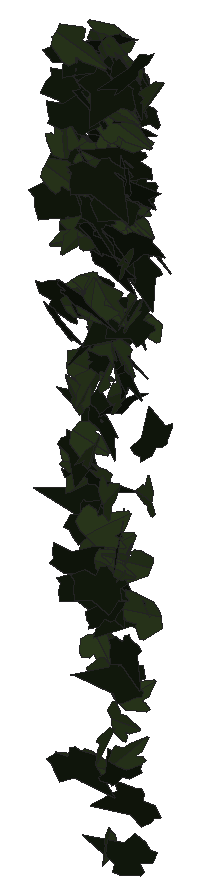
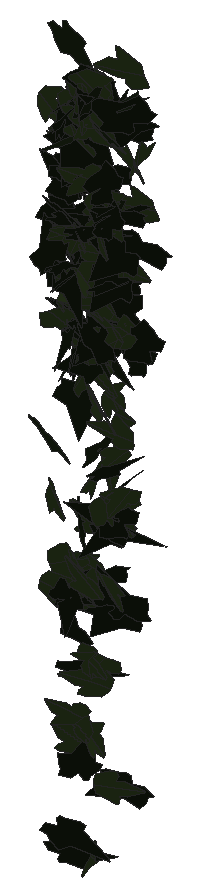
# SketchUp Ruby script. Lengths in inches.
U = 1.inch
M = Sketchup.active_model
def pt(a) = Geom::Point3d.new(a.map { |v| v * U })
def face(e, loops, mat)
  f = e.add_face(loops[0].map { |a| pt(a) })
  loops[1..].each { |l| e.add_face(l.map { |a| pt(a) }).erase! }
  f.material = f.back_material = mat if mat
  f
end
# faces: each face lists its corners as indices into pts; further lists are holes
def faces(e, pts, list, mat = nil) = list.each { |f| face(e, (f[0].is_a?(Array) ? f : [f]).map { |l| l.map { |i| pts[i] } }, mat) }
# xy, xz, yz: faces in a plane at the given z, y or x. An outline is a flat list of corners, or four numbers for a rectangle; further outlines are holes
def ring(l) = l.size == 4 ? [[l[0], l[1]], [l[2], l[1]], [l[2], l[3]], [l[0], l[3]]] : l.each_slice(2).to_a
def flat(e, list, mat, &to3) = list.each { |f| face(e, (f[0].is_a?(Array) ? f : [f]).map { |l| ring(l).map { |u, v| to3.(u, v) } }, mat) }
def xy(e, z, list, mat = nil) = flat(e, list, mat) { |x, y| [x, y, z] }
def xz(e, y, list, mat = nil) = flat(e, list, mat) { |x, z| [x, y, z] }
def yz(e, x, list, mat = nil) = flat(e, list, mat) { |y, z| [x, y, z] }
def lines(e, pts, list) = list.each { |a, b| e.add_line(pt(pts[a]), pt(pts[b])) }
# prism: a flat outline (further loops are holes) pulled along v
def prism(e, loops, v, mat = nil)
  f = face(e, loops, mat); d = Geom::Vector3d.new(v.map { |x| x * U })
  f.pushpull(f.normal.samedirection?(d) ? d.length : -d.length)
end
def box(e, o, s, mat = nil) = prism(e, [[o, [o[0] + s[0], o[1], o[2]], [o[0] + s[0], o[1] + s[1], o[2]], [o[0], o[1] + s[1], o[2]]]], [0, 0, s[2]], mat)
def at(x, y, z, deg = 0) = Geom::Transformation.translation(pt([x, y, z])) * Geom::Transformation.rotation(ORIGIN, Z_AXIS, deg.degrees)
def axes(o, x, y, z) = Geom::Transformation.new([*x, 0, *y, 0, *z, 0, *pt(o).to_a, 1])
def part(name) = M.definitions.add(name)
# library, detail: a bought-in or finely detailed component or shape, given as its bounding box
def library(name, o, s) = part(name).tap { |d| box(d.entities, o, s) }
def detail(e, o, s) = box(e.add_group.entities, o, s)
def put(e, d, t, mat = nil) = e.add_instance(d, t).tap { |i| i.material = mat if mat }
def group(e, t, mat = nil) = e.add_group.tap { |g| g.transformation = t; g.material = mat if mat }.entities
root = M.entities
M.materials.add("1026 AP 7946 SUNNY SIDE UP").color = [254, 231, 186]
M.materials.add("efeu1").color = [18, 25, 13]
M.materials.add("efeu2").color = [43, 57, 29]
c1 = part("ivyleaf_9")
p = [[1.54,2.16,1.25],[1.36,2.04,1.19],[-0.21,0.99,0.68],[-0.71,1.11,0.82],[-0.85,0.86,0.67],[-0.8,0.17,0.21],
  [-0.9,-0.01,0.1],[-0.67,-0.16,-0.02],[-0.08,-0.08,-0.05],[-0.03,-0.6,-0.4],[0.65,-0.88,-0.66],[0.83,-0.6,-0.49],
  [1.29,-0.42,-0.43],[1.8125,-0.07,-0.26],[1.21,0.44,0.15]]
faces(c1.entities,p,[[0,1,2,3,4,5,6,7,8,9,10,11,12,13,14]],"efeu1")
c2 = part("ivyleaf_10")
p = [[0,0.5,-0.03],[-0.0625,2.02,-0.43],[-0.19,2.01,-0.46],[-0.54,1.05,-0.29],[-0.52,0.625,-0.18],[-0.83,0.76,-0.28],
  [-1.16,0.64,-0.33],[-1.15,0.33,-0.24],[-0.77,-0.39,0.02],[-0.3,-0.51,0.16],[0.04,-0.48,0.23],[-0.02,2.01,-0.4375],
  [-0.06,2.01,-0.43],[0.04,-0.49,0.23],[0.67,-0.49,0.14],[1.38,0.36,-0.2],[1.375,0.51,-0.24],[0.81,0.65,-0.19],
  [0.62,0.59,-0.15],[0.6,1.09,-0.28],[0.5,1.23,-0.31]]
faces(c2.entities,p,[[0,1,2,3,4,5,6,7,8,9,10],[11,12,0,13,14,15,16,17,18,19,20]],"efeu2")
put(root,c1,axes([117.72,211.5625,267.85],[-0.26724,0.28496,-0.02816],[0.00004,-0.03365,-0.34156],[-0.45038,-0.16909,0.01668]),"1026 AP 7946 SUNNY SIDE UP")
put(root,c1,axes([116.79,211.63,257.41],[-0.02076,-0.2244,-0.18737],[0.03062,0.17968,-0.23041],[0.45189,-0.02249,0.00701]),"1026 AP 7946 SUNNY SIDE UP")
put(root,c2,axes([116.09,211.51,265.79],[-0.01025,0.27119,-0.1331],[-0.00358,0.13072,0.28022],[0.47338,0.00686,-0.00077]),"1026 AP 7946 SUNNY SIDE UP")
put(root,c1,axes([116.12,211.68,262.83],[0.32105,-0.12024,0.12963],[0.15877,-0.07745,-0.24415],[0.22386,0.22737,-0.01276]),"1026 AP 7946 SUNNY SIDE UP")
put(root,c2,axes([117.15,211.84,261.14],[-0.07556,0.10256,0.29182],[0.18442,-0.2572,0.11517],[0.43539,0.12674,0.00186]),"1026 AP 7946 SUNNY SIDE UP")
put(root,c2,axes([117.125,211.43,259.16],[0.0733,-0.01867,-0.30202],[0.03099,0.29626,-0.01448],[0.46071,-0.01696,0.04903]),"1026 AP 7946 SUNNY SIDE UP")
put(root,c1,axes([117.27,211.76,256.19],[-0.12056,-0.04186,-0.24779],[0.38238,0.00622,-0.08102],[0.02944,-0.25215,0.03762]),"1026 AP 7946 SUNNY SIDE UP")
put(root,c1,axes([116.625,211.8,264.67],[0.12053,-0.26928,0.01514],[-0.00287,-0.01738,-0.28845],[0.42417,0.0764,-0.00626]),"1026 AP 7946 SUNNY SIDE UP")
put(root,c1,axes([116.74,211.69,265.49],[-0.06701,-0.22295,-0.2213],[0.09219,0.20581,-0.23221],[0.47661,-0.07116,0.0138]),"1026 AP 7946 SUNNY SIDE UP")
put(root,c1,axes([116.25,211.62,266.28],[-0.25433,-0.035,0.20143],[0.29964,0.04473,0.17073],[-0.08923,0.24994,-0.00081]),"1026 AP 7946 SUNNY SIDE UP")
put(root,c1,axes([117.07,211.52,256.78],[-0.30564,0.1542,-0.11242],[-0.11394,0.08508,0.25529],[0.27517,0.2065,-0.01915]),"1026 AP 7946 SUNNY SIDE UP")
put(root,c2,axes([116.74,211.63,258.34],[0.32859,0.02524,-0.21949],[0.32306,0.0628,0.21549],[0.09792,-0.29186,0.02559]),"1026 AP 7946 SUNNY SIDE UP")
put(root,c1,axes([117.26,211.88,261.42],[0.01288,0.043,0.27915],[-0.13755,-0.25628,0.04316],[0.40849,-0.08765,0.00573]),"1026 AP 7946 SUNNY SIDE UP")
put(root,c2,axes([117.11,211.83,261.97],[-0.13057,0.05799,-0.24048],[0.22672,-0.18609,-0.10141],[-0.30335,-0.16404,0.02772]),"1026 AP 7946 SUNNY SIDE UP")
put(root,c2,axes([116.46,211.89,261.13],[-0.02177,-0.18039,0.2002],[0.07607,-0.19407,-0.18221],[0.41113,0.02636,0.04431]),"1026 AP 7946 SUNNY SIDE UP")
put(root,c1,axes([117.25,211.66,261.83],[0.26321,-0.14179,-0.16578],[-0.19682,0.09992,-0.22538],[0.27268,0.20898,-0.00265]),"1026 AP 7946 SUNNY SIDE UP")
put(root,c1,axes([117.39,211.66,264.42],[0.34811,0.14712,-0.16273],[-0.18976,-0.10467,-0.27386],[-0.28257,0.25154,-0.01656]),"1026 AP 7946 SUNNY SIDE UP")
put(root,c2,axes([115.73,211.74,265.09],[0.118,0.0225,0.25752],[0.39046,0.03029,-0.07948],[-0.05589,0.2591,-0.01152]),"1026 AP 7946 SUNNY SIDE UP")
put(root,c2,axes([116.88,211.87,254.21],[0.07301,-0.22861,0.12838],[0.04624,-0.12249,-0.241],[0.40777,0.05482,0.00434]),"1026 AP 7946 SUNNY SIDE UP")
put(root,c1,axes([115.6875,211.88,262.07],[0.13236,-0.1288,0.1951],[0.14711,-0.16568,-0.15928],[0.32975,0.12561,-0.00725]),"1026 AP 7946 SUNNY SIDE UP")
put(root,c1,axes([116.75,211.7,264.22],[0.41584,-0.01644,-0.15846],[-0.24309,-0.02609,-0.27128],[0.00162,0.30478,-0.02997]),"1026 AP 7946 SUNNY SIDE UP")
put(root,c1,axes([117.06,211.97,258.49],[-0.13244,0.00523,-0.31244],[0.40971,-0.15995,-0.07832],[-0.24427,-0.27112,0.03803]),"1026 AP 7946 SUNNY SIDE UP")
put(root,c1,axes([116.96,211.91,267.13],[-0.38473,-0.10593,-0.05945],[0.09598,0.00225,-0.27375],[0.16307,-0.25124,0.02088]),"1026 AP 7946 SUNNY SIDE UP")
put(root,c2,axes([117.38,211.86,264.01],[0.07415,-0.2657,0.03557],[0.0027,-0.03629,-0.27817],[0.42161,0.04696,-0.00447]),"1026 AP 7946 SUNNY SIDE UP")
put(root,c2,axes([116.57,211.76,262.6],[0.41928,-0.03942,0.02358],[-0.02972,0.02947,0.27653],[-0.06542,-0.26602,0.02553]),"1026 AP 7946 SUNNY SIDE UP")
put(root,c2,axes([116.38,211.72,260.71],[0.18063,-0.02954,0.22912],[-0.31798,0.09502,0.12107],[-0.1534,-0.23175,0.01883]),"1026 AP 7946 SUNNY SIDE UP")
put(root,c2,axes([115.94,211.82,267.76],[0.13322,0.02536,0.31168],[0.47296,0.03459,-0.0896],[-0.06324,0.31214,-0.01354]),"1026 AP 7946 SUNNY SIDE UP")
put(root,c1,axes([117.33,211.94,255.38],[-0.24724,-0.01,0.22267],[-0.32651,-0.06836,-0.15924],[0.09593,-0.25844,0.03188]),"1026 AP 7946 SUNNY SIDE UP")
put(root,c2,axes([116.74,211.9,257.58],[0.00141,-0.02321,-0.26083],[0.35543,-0.11553,0.01107],[-0.18254,-0.22514,0.01953]),"1026 AP 7946 SUNNY SIDE UP")
put(root,c1,axes([116.07,211.8,253.49],[-0.0324,-0.06753,-0.25995],[0.27629,0.18319,-0.06432],[0.30313,-0.17419,0.03084]),"1026 AP 7946 SUNNY SIDE UP")
put(root,c1,axes([117.2,212,256.84],[-0.34404,-0.14638,0.03912],[-0.02925,-0.04169,-0.27031],[0.23631,-0.21827,0.0235]),"1026 AP 7946 SUNNY SIDE UP")
put(root,c2,axes([116.7,211.875,262.91],[0.24586,0.01335,0.2242],[0.34266,-0.00423,-0.16111],[-0.00685,0.26788,-0.01214]),"1026 AP 7946 SUNNY SIDE UP")
put(root,c1,axes([117.11,211.93,253.45],[0.17044,0.1016,0.21229],[-0.27357,-0.11155,0.15071],[0.23471,-0.2038,0.0215]),"1026 AP 7946 SUNNY SIDE UP")
put(root,c2,axes([117.26,211.75,253.9],[-0.08504,-0.19327,0.17992],[0.04972,0.17331,0.20739],[-0.40774,0.06144,-0.01223]),"1026 AP 7946 SUNNY SIDE UP")
put(root,c2,axes([115.97,211.8,265.82],[0.3706,-0.14862,0.05043],[-0.04277,0.04978,0.28597],[-0.24271,-0.2357,0.02661]),"1026 AP 7946 SUNNY SIDE UP")
put(root,c2,axes([116.52,211.83,259.81],[-0.00742,-0.25742,-0.07225],[-0.00589,0.06874,-0.26479],[0.41889,-0.00359,-0.005]),"1026 AP 7946 SUNNY SIDE UP")
put(root,c1,axes([116.43,212.03,266.51],[0.22781,-0.24043,-0.04475],[0.05576,-0.02768,0.28855],[-0.37972,-0.14831,0.01552]),"1026 AP 7946 SUNNY SIDE UP")
put(root,c1,axes([115.6,211.92,262.4],[0.13012,-0.03081,0.27194],[0.34334,-0.15004,-0.08938],[0.23869,0.23261,-0.01968]),"1026 AP 7946 SUNNY SIDE UP")
put(root,c1,axes([116.41,211.71,258.5],[0.07428,-0.06146,-0.28555],[-0.10241,0.2708,-0.0718],[0.43398,0.07442,0.03193]),"1026 AP 7946 SUNNY SIDE UP")
put(root,c1,axes([116.95,212.07,262.44],[-0.28264,-0.16476,0.10937],[-0.09794,-0.0899,-0.25068],[0.29306,-0.18894,0.02171]),"1026 AP 7946 SUNNY SIDE UP")
put(root,c2,axes([116.29,212.02,263.91],[-0.12306,-0.08708,0.25223],[-0.23051,-0.19695,-0.12135],[0.33826,-0.16589,0.00907]),"1026 AP 7946 SUNNY SIDE UP")
put(root,c2,axes([116.65,211.89,266.75],[-0.1529,-0.02439,-0.2596],[0.39621,-0.03393,-0.09704],[-0.03627,-0.26784,0.03433]),"1026 AP 7946 SUNNY SIDE UP")
put(root,c2,axes([117.73,211.88,256.91],[0.13006,-0.04594,-0.314],[-0.46932,0.0658,-0.09335],[0.11941,0.30863,-0.02491]),"1026 AP 7946 SUNNY SIDE UP")
put(root,c1,axes([116.08,212.08,259.54],[-0.05059,-0.23355,0.11083],[-0.0225,-0.10796,-0.24351],[0.40458,-0.03521,0.00032]),"1026 AP 7946 SUNNY SIDE UP")
put(root,c1,axes([116.8,211.85,263.66],[0.41958,-0.01822,-0.04938],[-0.07755,-0.02367,-0.27432],[0.02151,0.27006,-0.02578]),"1026 AP 7946 SUNNY SIDE UP")
put(root,c1,axes([116.99,212.1,264.8125],[-0.31863,-0.13902,0.12709],[-0.12632,-0.10034,-0.25141],[0.26445,-0.21543,0.03303]),"1026 AP 7946 SUNNY SIDE UP")
put(root,c2,axes([116.23,212.07,264.02],[-0.14356,-0.20582,0.20349],[-0.055,-0.19897,-0.23005],[0.44645,-0.09069,0.03709]),"1026 AP 7946 SUNNY SIDE UP")
put(root,c1,axes([117.49,211.98,262.64],[-0.44547,0.07154,0.0402],[-0.06956,-0.01819,-0.29972],[-0.10725,-0.28535,0.0274]),"1026 AP 7946 SUNNY SIDE UP")
put(root,c2,axes([117.29,211.93,262.91],[0.14995,-0.28821,-0.04371],[-0.03315,0.03597,-0.31241],[0.4565,0.09728,-0.00833]),"1026 AP 7946 SUNNY SIDE UP")
put(root,c2,axes([116.5,211.97,253.39],[-0.03007,-0.02828,-0.25628],[-0.39185,-0.02019,0.022],[-0.03525,0.24853,-0.0259]),"1026 AP 7946 SUNNY SIDE UP")
put(root,c1,axes([116.51,212,258.59],[-0.19568,-0.11121,-0.24194],[-0.31265,-0.12579,0.16964],[-0.26164,0.23349,-0.02177]),"1026 AP 7946 SUNNY SIDE UP")
put(root,c1,axes([116.57,212.01,262.14],[-0.30919,0.16397,-0.16959],[0.17322,-0.12545,-0.26355],[-0.32285,-0.22435,0.021]),"1026 AP 7946 SUNNY SIDE UP")
put(root,c1,axes([117.125,212,265.14],[0.3503,0.00581,-0.12442],[0.18747,0.03202,0.22827],[0.03197,-0.2514,0.0247]),"1026 AP 7946 SUNNY SIDE UP")
put(root,c1,axes([115.97,212.09,266.76],[-0.13009,-0.30235,-0.04442],[0.02303,0.03892,-0.32268],[0.4793,-0.08394,0.00345]),"1026 AP 7946 SUNNY SIDE UP")
put(root,c2,axes([117.38,211.8,262.61],[0.18968,-0.13147,0.21383],[-0.10355,0.2063,0.17462],[-0.37323,-0.12404,0.06023]),"1026 AP 7946 SUNNY SIDE UP")
put(root,c1,axes([117.16,211.83,260.93],[0.06938,0.26889,0.0308],[0.0143,0.02726,-0.28051],[-0.42491,0.04482,-0.00441]),"1026 AP 7946 SUNNY SIDE UP")
put(root,c2,axes([116.29,211.82,259.99],[0.04098,0.19108,0.2103],[0.06181,0.19938,-0.19732],[-0.43404,0.04643,-0.00825]),"1026 AP 7946 SUNNY SIDE UP")
put(root,c1,axes([115.67,212,264.54],[-0.09109,-0.1482,-0.29127],[0.34846,0.18702,-0.14711],[0.35965,-0.21873,0.06876]),"1026 AP 7946 SUNNY SIDE UP")
put(root,c2,axes([116.68,212.14,251.97],[-0.00617,0.15818,-0.20222],[-0.0059,-0.19723,-0.16406],[-0.39745,0.00047,0.00557]),"1026 AP 7946 SUNNY SIDE UP")
put(root,c2,axes([117.375,212.14,257.64],[-0.07896,-0.03949,-0.26284],[-0.34876,-0.12598,0.06438],[-0.20709,0.22722,-0.0082]),"1026 AP 7946 SUNNY SIDE UP")
put(root,c2,axes([117.03,211.98,257.44],[0.17186,-0.23337,0.06481],[-0.02728,0.06274,0.26562],[-0.37961,-0.11016,0.01025]),"1026 AP 7946 SUNNY SIDE UP")
put(root,c1,axes([116.19,212.01,256.95],[-0.11414,-0.15226,-0.2073],[0.15421,0.17493,-0.17252],[0.36441,-0.12171,0.00808]),"1026 AP 7946 SUNNY SIDE UP")
put(root,c2,axes([116.67,211.89,255.31],[-0.08783,-0.06651,0.25795],[0.23571,0.20109,0.09051],[-0.33295,0.1599,-0.00397]),"1026 AP 7946 SUNNY SIDE UP")
put(root,c1,axes([117.23,211.89,265.22],[0.0127,-0.05805,0.26749],[-0.03698,0.25893,0.06183],[-0.41723,-0.02472,0.00266]),"1026 AP 7946 SUNNY SIDE UP")
put(root,c2,axes([116.53,212,255.88],[0.31304,0.14071,0.10499],[0.1511,0.0385,-0.24989],[-0.22672,0.21995,-0.02158]),"1026 AP 7946 SUNNY SIDE UP")
put(root,c1,axes([117.36,212.0625,251.76],[-0.12208,0.04315,0.24752],[-0.37833,0.0275,-0.08511],[-0.0625,-0.25076,0.03173]),"1026 AP 7946 SUNNY SIDE UP")
put(root,c2,axes([116.86,212.08,254.38],[-0.12894,0.04516,0.24159],[0.36301,-0.04743,0.0924],[0.09457,0.24362,-0.02527]),"1026 AP 7946 SUNNY SIDE UP")
put(root,c2,axes([116.79,212.01,266.39],[0.18016,0.06357,0.28632],[0.42571,0.06839,-0.13087],[-0.13875,0.2924,-0.02976]),"1026 AP 7946 SUNNY SIDE UP")
put(root,c2,axes([116.73,212.03,262.41],[-0.42766,-0.01177,0.14333],[-0.2149,-0.04059,-0.27888],[0.04543,-0.30282,0.03]),"1026 AP 7946 SUNNY SIDE UP")
put(root,c2,axes([116.3,212.14,259.12],[-0.26657,-0.17668,0.17148],[-0.15761,-0.13529,-0.25239],[0.34881,-0.19616,0.01701]),"1026 AP 7946 SUNNY SIDE UP")
put(root,c1,axes([116,212.05,257.08],[-0.22633,0.01174,0.24378],[0.3247,-0.12938,0.13529],[0.18243,0.24484,0.06164]),"1026 AP 7946 SUNNY SIDE UP")
put(root,c2,axes([116.08,211.91,262.47],[-0.07267,-0.08747,0.25326],[0.1854,0.21628,0.10317],[-0.36684,0.12664,0.00198]),"1026 AP 7946 SUNNY SIDE UP")
put(root,c1,axes([116.42,212.22,260.2],[0.09194,-0.23113,0.09239],[0.0245,-0.08988,-0.24605],[0.38981,0.06016,-0.00632]),"1026 AP 7946 SUNNY SIDE UP")
put(root,c1,axes([116.2,212.24,266.98],[0.06528,-0.26269,0.06595],[0.00886,-0.06542,-0.27433],[0.42561,0.04165,-0.0044]),"1026 AP 7946 SUNNY SIDE UP")
put(root,c2,axes([117.42,212.16,262.54],[0.30132,0.0458,-0.1741],[-0.25436,-0.05054,-0.20307],[-0.10636,0.25063,-0.00757]),"1026 AP 7946 SUNNY SIDE UP")
put(root,c1,axes([117.25,212.05,257.06],[0.29601,-0.03826,-0.19413],[-0.29965,-0.00424,-0.19549],[0.03778,0.26618,-0.02943]),"1026 AP 7946 SUNNY SIDE UP")
put(root,c1,axes([115.94,212.34,267.25],[-0.21248,-0.17848,0.173],[0.01144,-0.19562,-0.20805],[0.38626,-0.09239,0.10133]),"1026 AP 7946 SUNNY SIDE UP")
put(root,c2,axes([116.91,212,255.84],[0.05367,-0.0373,-0.26887],[-0.28418,0.188,-0.05097],[0.30137,0.18392,-0.00018]),"1026 AP 7946 SUNNY SIDE UP")
put(root,c1,axes([117.25,212.2,265.62],[-0.17938,-0.01174,-0.23279],[-0.2336,-0.1869,0.0862],[-0.26823,0.17062,0.08061]),"1026 AP 7946 SUNNY SIDE UP")
put(root,c1,axes([116.64,212.14,267.26],[0.32328,-0.16516,-0.03346],[-0.04727,0.01291,-0.27146],[0.26013,0.2076,-0.00774]),"1026 AP 7946 SUNNY SIDE UP")
put(root,c1,axes([116.02,212.09,258.84],[0.17235,-0.02215,0.241],[0.3632,-0.03801,-0.11536],[0.06893,0.25564,0.00527]),"1026 AP 7946 SUNNY SIDE UP")
put(root,c1,axes([116.54,212.17,261.9375],[0.34666,-0.14483,0.07411],[0.07705,-0.05753,-0.27127],[0.24293,0.22492,-0.01971]),"1026 AP 7946 SUNNY SIDE UP")
put(root,c2,axes([117,212.11,266.03],[0.44621,-0.03109,-0.01243],[0.02322,0.02614,0.29287],[-0.04691,-0.28282,0.02674]),"1026 AP 7946 SUNNY SIDE UP")
put(root,c2,axes([116.5,212.17,260.99],[0.2054,-0.22767,0.0194],[0.00207,0.02393,0.27022],[-0.35938,-0.12998,0.01264]),"1026 AP 7946 SUNNY SIDE UP")
put(root,c1,axes([117.2,212.26,263.56],[-0.20615,-0.06285,-0.2308],[0.34581,0.04928,-0.14677],[0.11785,-0.25455,0.02694]),"1026 AP 7946 SUNNY SIDE UP")
put(root,c2,axes([116.06,212.27,262.65],[0.09208,-0.06387,-0.25473],[0.32897,-0.13283,0.08574],[-0.22932,-0.21621,0.02072]),"1026 AP 7946 SUNNY SIDE UP")
put(root,c2,axes([116.64,212.16,261.82],[0.26996,-0.06793,-0.19761],[-0.25824,0.10108,-0.1881],[0.18797,0.23644,0.02539]),"1026 AP 7946 SUNNY SIDE UP")
put(root,c2,axes([116.625,212.22,264.14],[-0.04457,-0.02312,-0.25791],[-0.39498,0.00921,0.02849],[0.01037,0.25165,-0.02326]),"1026 AP 7946 SUNNY SIDE UP")
put(root,c1,axes([116.06,212.35,265.11],[0.18491,-0.22094,0.14796],[0.10406,-0.12889,-0.25859],[0.40219,0.13493,-0.00112]),"1026 AP 7946 SUNNY SIDE UP")
put(root,c1,axes([116.78,212.08,266.2],[0.38203,0.18049,-0.03085],[-0.01681,-0.03738,-0.31108],[-0.28746,0.24205,-0.0228]),"1026 AP 7946 SUNNY SIDE UP")
put(root,c1,axes([115.86,212.38,265.21],[-0.10986,-0.29429,0.00657],[0.00951,-0.0097,-0.31155],[0.46282,-0.06966,0.00796]),"1026 AP 7946 SUNNY SIDE UP")
put(root,c1,axes([116.44,212.08,262.51],[0.29711,0.16785,0.03664],[0.06185,0.00767,-0.25949],[-0.26229,0.19194,-0.01969]),"1026 AP 7946 SUNNY SIDE UP")
put(root,c2,axes([116.24,212.26,257.7],[0.32072,-0.14378,-0.06943],[-0.09674,0.02814,-0.25662],[0.2296,0.2127,-0.01115]),"1026 AP 7946 SUNNY SIDE UP")
put(root,c2,axes([115.85,212.17,259.52],[0.16167,0.22006,0.10697],[0.07181,0.09188,-0.24968],[-0.37495,0.11248,-0.0017]),"1026 AP 7946 SUNNY SIDE UP")
put(root,c1,axes([116.88,212.39,267.22],[0.07401,-0.26946,0.0409],[0.00274,-0.04155,-0.28199],[0.42863,0.04679,-0.00526]),"1026 AP 7946 SUNNY SIDE UP")
put(root,c2,axes([116.31,212.36,265.35],[-0.22477,-0.06744,0.19727],[-0.20315,-0.15101,-0.15473],[0.24698,-0.18559,0.05226]),"1026 AP 7946 SUNNY SIDE UP")
put(root,c2,axes([116.19,212.29,264.95],[-0.34794,0.0296,-0.11484],[0.16278,-0.05619,-0.22705],[-0.08056,-0.2414,0.03725]),"1026 AP 7946 SUNNY SIDE UP")
put(root,c1,axes([117.25,212.45,263.88],[0.34805,-0.13106,-0.14432],[0.20936,-0.04745,0.2636],[-0.21597,-0.25722,0.02296]),"1026 AP 7946 SUNNY SIDE UP")
put(root,c1,axes([116.88,212.33,263.8],[-0.09997,-0.22355,-0.13765],[0.07015,0.12483,-0.23857],[0.40242,-0.0773,0.00739]),"1026 AP 7946 SUNNY SIDE UP")
put(root,c2,axes([116.89,212.23,264.47],[0.22207,0.0759,0.20327],[0.26785,0.0988,-0.16454],[-0.1958,0.22124,0.00545]),"1026 AP 7946 SUNNY SIDE UP")
put(root,c2,axes([116.39,212.3,267.7],[-0.37014,0.07903,-0.06136],[0.07478,-0.04575,-0.25451],[-0.13695,-0.23858,0.02688]),"1026 AP 7946 SUNNY SIDE UP")
put(root,c2,axes([115.94,212.2,262.66],[0.17326,0.16311,0.1789],[0.17216,0.13412,-0.20164],[-0.33154,0.15489,-0.01121]),"1026 AP 7946 SUNNY SIDE UP")
put(root,c2,axes([116.86,212.13,262.33],[0.04965,-0.1195,-0.25432],[-0.02277,0.24675,-0.12385],[0.4297,0.02688,0.02283]),"1026 AP 7946 SUNNY SIDE UP")
put(root,c1,axes([116.07,212.39,265.63],[0.2063,-0.13117,0.1929],[0.20367,-0.13629,-0.19189],[0.29739,0.18433,-0.0024]),"1026 AP 7946 SUNNY SIDE UP")
put(root,c2,axes([117.55,212.17,258.99],[-0.07242,0.06233,0.2697],[-0.35352,0.13641,-0.07351],[-0.23157,-0.22774,0.02787]),"1026 AP 7946 SUNNY SIDE UP")
put(root,c2,axes([116.76,212.3,264.48],[0.31674,0.16176,0.06429],[0.09585,0.02198,-0.26519],[-0.25467,0.20946,-0.01985]),"1026 AP 7946 SUNNY SIDE UP")
put(root,c1,axes([117.07,212.47,264.75],[-0.3457,-0.0441,0.14967],[-0.20946,-0.06755,-0.22879],[0.11534,-0.25486,0.0331]),"1026 AP 7946 SUNNY SIDE UP")
put(root,c1,axes([116.82,212.54,267.21],[-0.08321,-0.25514,0.10483],[-0.02255,-0.1024,-0.26896],[0.43218,-0.05446,0.00615]),"1026 AP 7946 SUNNY SIDE UP")
put(root,c1,axes([117.02,212.28,262.45],[0.25496,-0.12269,-0.17691],[-0.24466,0.07552,-0.20735],[0.22289,0.22325,-0.02524]),"1026 AP 7946 SUNNY SIDE UP")
put(root,c2,axes([117.42,212.48,267.01],[0.02513,-0.24072,0.13063],[0.00921,-0.12806,-0.24927],[0.42872,0.01686,-0.00231]),"1026 AP 7946 SUNNY SIDE UP")
put(root,c1,axes([117.65,212.18,260.125],[-0.32907,0.10499,-0.18374],[-0.22859,0.10714,0.24053],[0.23276,0.25366,-0.02354]),"1026 AP 7946 SUNNY SIDE UP")
put(root,c1,axes([115.69,212.24,267.06],[-0.07295,0.02582,0.30671],[0.46155,0.05968,0.04216],[-0.08694,0.2952,-0.03354]),"1026 AP 7946 SUNNY SIDE UP")
put(root,c2,axes([117.05,212.36,263.47],[0.02981,-0.03503,-0.27113],[-0.4019,0.06828,-0.02795],[0.11185,0.25467,-0.02817]),"1026 AP 7946 SUNNY SIDE UP")
put(root,c2,axes([116.91,212.27,254.79],[0.21735,0.06666,-0.2084],[0.25602,0.1231,0.15683],[0.2168,-0.2122,0.02373]),"1026 AP 7946 SUNNY SIDE UP")
put(root,c2,axes([116.3125,212.48,266.83],[0.26421,0.15205,-0.14449],[-0.15262,-0.10288,-0.23385],[-0.28828,0.19382,-0.00862]),"1026 AP 7946 SUNNY SIDE UP")
put(root,c2,axes([116.41,212.43,257.51],[0.32197,-0.11278,-0.1815],[0.26071,-0.06135,0.23949],[-0.19916,-0.26263,0.02009]),"1026 AP 7946 SUNNY SIDE UP")
put(root,c1,axes([116.15,212.46,262.63],[0.07906,-0.02604,-0.27905],[0.42259,0.04699,0.04704],[0.0656,-0.27131,0.03327]),"1026 AP 7946 SUNNY SIDE UP")
put(root,c1,axes([116.32,212.49,266.95],[-0.33471,0.08113,-0.10957],[0.13075,-0.07741,-0.23172],[-0.1655,-0.22523,0.03853]),"1026 AP 7946 SUNNY SIDE UP")
put(root,c2,axes([116.63,212.24,265.58],[0.1673,0.0999,-0.25657],[0.25234,0.19179,0.15067],[0.3392,-0.19195,0.01447]),"1026 AP 7946 SUNNY SIDE UP")
put(root,c1,axes([115.76,212.43,265.3],[-0.07282,-0.17292,-0.19153],[0.16241,0.15874,-0.17863],[0.36347,-0.10557,0.04144]),"1026 AP 7946 SUNNY SIDE UP")
put(root,c2,axes([116.65,212.53,264.66],[0.17961,-0.19317,0.10874],[0.09388,-0.08856,-0.23164],[0.33403,0.12876,0.00663]),"1026 AP 7946 SUNNY SIDE UP")
put(root,c2,axes([116.52,212.53,267.72],[-0.27785,-0.08595,0.19537],[-0.22977,-0.12688,-0.19974],[0.2342,-0.22644,0.03583]),"1026 AP 7946 SUNNY SIDE UP")
put(root,c1,axes([116.38,212.3125,267.66],[0.21989,0.21718,0.01606],[0.02702,0.006,-0.26582],[-0.34117,0.14045,-0.0107]),"1026 AP 7946 SUNNY SIDE UP")
put(root,c1,axes([115.83,212.29,264.42],[0.26048,0.17769,0.09012],[0.10691,0.05469,-0.24966],[-0.29176,0.17869,-0.01103]),"1026 AP 7946 SUNNY SIDE UP")
put(root,c1,axes([117.11,212.55,264.99],[-0.39654,0.03106,-0.08604],[0.12481,-0.03673,-0.26067],[-0.06422,-0.26316,0.02464]),"1026 AP 7946 SUNNY SIDE UP")
put(root,c1,axes([116.31,212.3,261.1],[-0.02943,0.12504,0.22923],[-0.09597,0.21372,-0.12817],[-0.3887,-0.06223,0.01429]),"1026 AP 7946 SUNNY SIDE UP")
put(root,c1,axes([116.99,212.625,266.6],[-0.05593,0.03435,0.25511],[-0.00797,-0.24998,0.03353],[0.39272,-0.00018,0.03701]),"1026 AP 7946 SUNNY SIDE UP")
put(root,c1,axes([116.65,212.6,264.63],[-0.24554,0.0068,0.20224],[-0.28962,-0.0921,-0.14821],[0.10717,-0.2333,0.06283]),"1026 AP 7946 SUNNY SIDE UP")
put(root,c2,axes([116.77,212.5,267.28],[-0.32576,0.01532,0.15626],[-0.23718,-0.05677,-0.20679],[0.03384,-0.25036,0.05491]),"1026 AP 7946 SUNNY SIDE UP")
put(root,c1,axes([115.79,212.52,263.86],[-0.04536,-0.22278,-0.14936],[0.07459,0.13789,-0.22921],[0.41013,-0.04971,0.02517]),"1026 AP 7946 SUNNY SIDE UP")
put(root,c1,axes([116.74,212.59,263.76],[0.09551,-0.26212,-0.03405],[-0.01399,0.03034,-0.277],[0.4149,0.06136,-0.0015]),"1026 AP 7946 SUNNY SIDE UP")
put(root,c1,axes([116.12,212.625,260.02],[-0.12557,-0.22987,-0.06338],[-0.0234,-0.05856,0.2503],[-0.37292,0.08108,0.00564]),"1026 AP 7946 SUNNY SIDE UP")
put(root,c2,axes([115.63,212.5,260.88],[-0.00722,0.02669,0.27014],[0.4068,0.04984,-0.00027],[-0.07804,0.25733,-0.02639]),"1026 AP 7946 SUNNY SIDE UP")
put(root,c1,axes([117.02,212.56,252.63],[-0.01958,0.00741,-0.26395],[-0.2977,-0.17325,0.0033],[-0.2718,0.18923,0.0154]),"1026 AP 7946 SUNNY SIDE UP")
put(root,c2,axes([116.38,212.42,264.79],[-0.20126,0.10947,0.2115],[-0.30256,0.08068,-0.16794],[-0.20413,-0.22752,0.0404]),"1026 AP 7946 SUNNY SIDE UP")
put(root,c1,axes([116.9375,212.46,263.62],[0.21533,-0.02516,-0.25017],[-0.38336,-0.02512,-0.13919],[-0.01518,0.27753,-0.03363]),"1026 AP 7946 SUNNY SIDE UP")
put(root,c1,axes([115.86,212.45,263.97],[0.39914,0.03199,-0.06199],[-0.08937,-0.02991,-0.26277],[-0.05958,0.2592,-0.02111]),"1026 AP 7946 SUNNY SIDE UP")
put(root,c2,axes([116.53,212.47,267.27],[-0.05849,-0.24285,-0.11232],[0.02387,0.10658,-0.25247],[0.417,-0.04016,-0.0013]),"1026 AP 7946 SUNNY SIDE UP")
put(root,c2,axes([116.35,212.55,267.04],[-0.33199,-0.19775,0.03862],[0.02429,0.03988,0.29765],[-0.31588,0.2109,-0.01771]),"1026 AP 7946 SUNNY SIDE UP")
put(root,c1,axes([116.92,212.75,266.375],[-0.17691,-0.17845,0.13921],[0.01129,-0.15507,-0.2042],[0.35275,-0.08453,0.07635]),"1026 AP 7946 SUNNY SIDE UP")
put(root,c1,axes([115.8,212.68,265.1],[0.07812,-0.08823,0.24273],[0.18723,-0.2039,-0.10549],[0.34933,0.12901,0.00226]),"1026 AP 7946 SUNNY SIDE UP")
put(root,c1,axes([116.93,212.53,266.72],[-0.17926,-0.21581,0.14195],[0.11297,0.11921,0.25204],[-0.38752,0.13458,0.00781]),"1026 AP 7946 SUNNY SIDE UP")
put(root,c1,axes([116.29,212.66,267.4375],[0.19509,-0.19759,0.10812],[0.08755,-0.09029,-0.24089],[0.34159,0.13599,-0.00001]),"1026 AP 7946 SUNNY SIDE UP")
put(root,c2,axes([116.41,212.6875,263.93],[0.07414,-0.22846,0.12929],[0.04627,-0.12338,-0.24102],[0.40824,0.05547,0.00384]),"1026 AP 7946 SUNNY SIDE UP")
